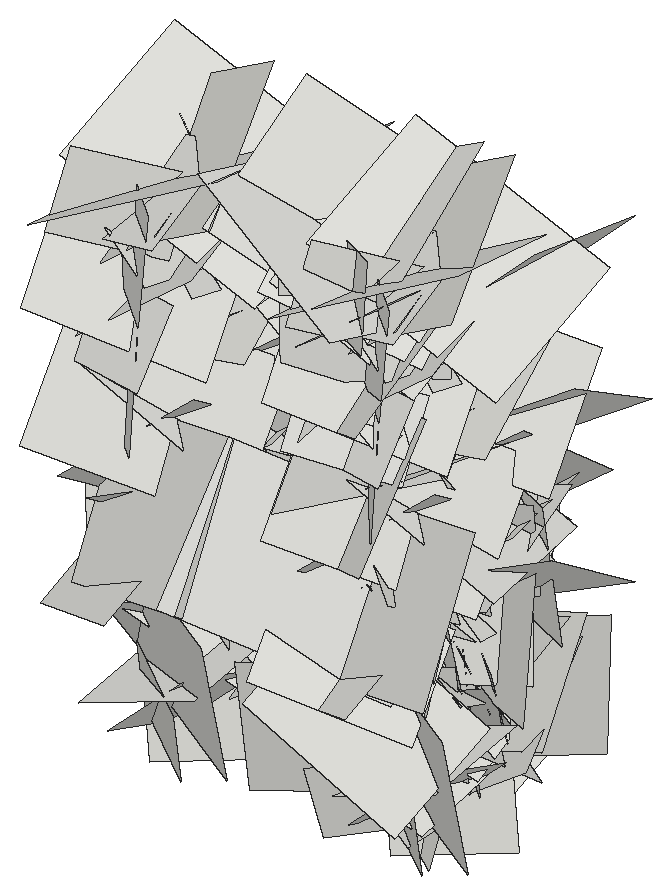
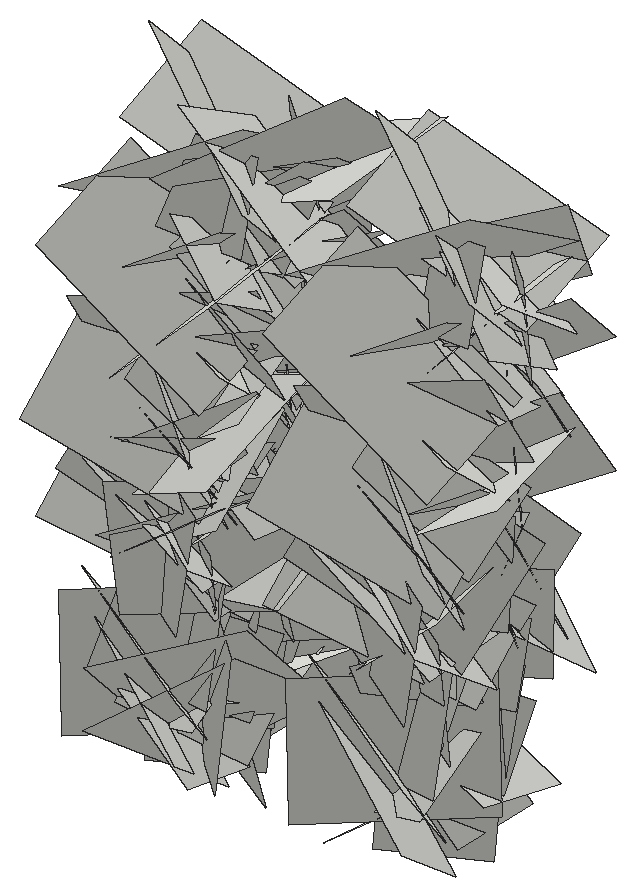
# SketchUp Ruby script. Lengths in inches.
U = 1.inch
M = Sketchup.active_model
def pt(a) = Geom::Point3d.new(a.map { |v| v * U })
def face(e, loops, mat)
  f = e.add_face(loops[0].map { |a| pt(a) })
  loops[1..].each { |l| e.add_face(l.map { |a| pt(a) }).erase! }
  f.material = f.back_material = mat if mat
  f
end
# faces: each face lists its corners as indices into pts; further lists are holes
def faces(e, pts, list, mat = nil) = list.each { |f| face(e, (f[0].is_a?(Array) ? f : [f]).map { |l| l.map { |i| pts[i] } }, mat) }
# xy, xz, yz: faces in a plane at the given z, y or x. An outline is a flat list of corners, or four numbers for a rectangle; further outlines are holes
def ring(l) = l.size == 4 ? [[l[0], l[1]], [l[2], l[1]], [l[2], l[3]], [l[0], l[3]]] : l.each_slice(2).to_a
def flat(e, list, mat, &to3) = list.each { |f| face(e, (f[0].is_a?(Array) ? f : [f]).map { |l| ring(l).map { |u, v| to3.(u, v) } }, mat) }
def xy(e, z, list, mat = nil) = flat(e, list, mat) { |x, y| [x, y, z] }
def xz(e, y, list, mat = nil) = flat(e, list, mat) { |x, z| [x, y, z] }
def yz(e, x, list, mat = nil) = flat(e, list, mat) { |y, z| [x, y, z] }
def lines(e, pts, list) = list.each { |a, b| e.add_line(pt(pts[a]), pt(pts[b])) }
# prism: a flat outline (further loops are holes) pulled along v
def prism(e, loops, v, mat = nil)
  f = face(e, loops, mat); d = Geom::Vector3d.new(v.map { |x| x * U })
  f.pushpull(f.normal.samedirection?(d) ? d.length : -d.length)
end
def box(e, o, s, mat = nil) = prism(e, [[o, [o[0] + s[0], o[1], o[2]], [o[0] + s[0], o[1] + s[1], o[2]], [o[0], o[1] + s[1], o[2]]]], [0, 0, s[2]], mat)
def at(x, y, z, deg = 0) = Geom::Transformation.translation(pt([x, y, z])) * Geom::Transformation.rotation(ORIGIN, Z_AXIS, deg.degrees)
def axes(o, x, y, z) = Geom::Transformation.new([*x, 0, *y, 0, *z, 0, *pt(o).to_a, 1])
def part(name) = M.definitions.add(name)
# library, detail: a bought-in or finely detailed component or shape, given as its bounding box
def library(name, o, s) = part(name).tap { |d| box(d.entities, o, s) }
def detail(e, o, s) = box(e.add_group.entities, o, s)
def put(e, d, t, mat = nil) = e.add_instance(d, t).tap { |i| i.material = mat if mat }
def group(e, t, mat = nil) = e.add_group.tap { |g| g.transformation = t; g.material = mat if mat }.entities
root = M.entities
c1 = part("Component\#6")
p = [[0.01,0,0],[0,3.24,4.54],[4.32,3.24,4.54],[4.33,0,0]]
faces(c1.entities,p,[[0,1,2,3]])
put(root,c1,axes([34.14,170.9375,7.01],[0.11124,0.9843,0.53665],[-0.15751,0.54645,-0.97322],[1.17787,-0.01989,-0.18083]))
put(root,c1,axes([24.34,177.17,11.87],[0.09089,-0.73345,-1.16692],[0.11565,-1.16189,0.73831],[1.45639,0.13804,0.0142]))
put(root,c1,axes([38.11,177.17,11.87],[-0.09089,-0.73345,-1.16692],[-0.11565,-1.16189,0.73831],[-1.45639,0.13804,0.0142]))
put(root,c1,axes([34.14,177.17,11.87],[0.09089,-0.73345,-1.16692],[0.11565,-1.16189,0.73831],[1.45639,0.13804,0.0142]))
put(root,c1,axes([28.31,171.15,7.72],[0.19789,0.75168,0.59634],[-0.00491,0.60823,-0.76521],[-1.01706,0.14332,0.11972]))
put(root,c1,axes([34.14,171.15,7.72],[-0.19789,0.75168,0.59634],[0.00491,0.60823,-0.76521],[1.01706,0.14332,0.11972]))
put(root,c1,axes([38.11,171.15,7.72],[0.19789,0.75168,0.59634],[-0.00491,0.60823,-0.76521],[-1.01706,0.14332,0.11972]))
put(root,c1,axes([28.31,175.79,22.11],[-0.09057,-0.18477,-0.67682],[0.07729,-0.68047,0.17656],[-0.73966,-0.04848,0.10132]))
put(root,c1,axes([34.14,175.79,22.11],[0.09057,-0.18477,-0.67682],[-0.07729,-0.68047,0.17656],[0.73966,-0.04848,0.10132]))
put(root,c1,axes([38.11,175.79,22.11],[-0.09057,-0.18477,-0.67682],[0.07729,-0.68047,0.17656],[-0.73966,-0.04848,0.10132]))
put(root,c1,axes([28.31,172.87,15.39],[0.04258,0.36909,0.59744],[-0.18529,0.58484,-0.34955],[-0.72096,-0.1285,0.12512]))
put(root,c1,axes([34.14,172.87,15.39],[-0.04258,0.36909,0.59744],[0.18529,0.58484,-0.34955],[0.72096,-0.1285,0.12512]))
put(root,c1,axes([38.11,172.87,15.39],[0.04258,0.36909,0.59744],[-0.18529,0.58484,-0.34955],[-0.72096,-0.1285,0.12512]))
put(root,c1,axes([24.34,176.71,20],[0.1716,-1.2405,0.25629],[0.15029,0.2745,1.23906],[1.33426,0.12862,-0.17253]))
put(root,c1,axes([38.11,176.71,20],[-0.1716,-1.2405,0.25629],[-0.15029,0.2745,1.23906],[-1.33426,0.12862,-0.17253]))
put(root,c1,axes([34.14,176.71,20],[0.1716,-1.2405,0.25629],[0.15029,0.2745,1.23906],[1.33426,0.12862,-0.17253]))
put(root,c1,axes([28.31,172.9,17.79],[0.05847,0.04666,0.93522],[0.13105,0.92828,-0.05361],[-0.98388,0.12642,0.04844]))
put(root,c1,axes([34.14,172.9,17.79],[-0.05847,0.04666,0.93522],[-0.13105,0.92828,-0.05361],[0.98388,0.12642,0.04844]))
put(root,c1,axes([38.11,172.9,17.79],[0.05847,0.04666,0.93522],[0.13105,0.92828,-0.05361],[-0.98388,0.12642,0.04844]))
put(root,c1,axes([28.31,172.44,13.26],[-0.14239,0.27787,0.83247],[0.25689,0.82117,-0.23499],[-0.89411,0.19168,-0.20009]))
put(root,c1,axes([34.14,172.44,13.26],[0.14239,0.27787,0.83247],[-0.25689,0.82117,-0.23499],[0.89411,0.19168,-0.20009]))
put(root,c1,axes([38.11,172.44,13.26],[-0.14239,0.27787,0.83247],[0.25689,0.82117,-0.23499],[-0.89411,0.19168,-0.20009]))
put(root,c1,axes([28.31,178.76,18.36],[0.19902,-0.79911,-0.76231],[0.1591,-0.74761,0.82067],[-1.1598,-0.23968,-0.01823]))
put(root,c1,axes([34.14,178.76,18.36],[-0.19902,-0.79911,-0.76231],[-0.1591,-0.74761,0.82067],[1.1598,-0.23968,-0.01823]))
put(root,c1,axes([38.11,178.76,18.36],[0.19902,-0.79911,-0.76231],[0.1591,-0.74761,0.82067],[-1.1598,-0.23968,-0.01823]))
put(root,c1,axes([24.34,178.02,21.625],[-0.10055,-0.80704,-0.57155],[0.14009,-0.57937,0.79615],[1.03886,0.00001,-0.16268]))
put(root,c1,axes([38.11,178.02,21.625],[0.10055,-0.80704,-0.57155],[-0.14009,-0.57937,0.79615],[-1.03886,0.00001,-0.16268]))
put(root,c1,axes([34.14,178.02,21.625],[-0.10055,-0.80704,-0.57155],[0.14009,-0.57937,0.79615],[1.03886,0.00001,-0.16268]))
put(root,c1,axes([24.34,171.875,12.53],[-0.03767,0.74177,1.03266],[-0.14299,1.02503,-0.74093],[1.34014,0.13022,-0.05004]))
put(root,c1,axes([38.11,171.875,12.53],[0.03767,0.74177,1.03266],[0.14299,1.02503,-0.74093],[-1.34014,0.13022,-0.05004]))
put(root,c1,axes([34.14,171.875,12.53],[-0.03767,0.74177,1.03266],[-0.14299,1.02503,-0.74093],[1.34014,0.13022,-0.05004]))
put(root,c1,axes([28.31,176.92,18.36],[-0.03591,-0.7978,0.13647],[0.05211,0.13431,0.79737],[-0.85636,0.04162,0.0428]))
put(root,c1,axes([34.14,176.92,18.36],[0.03591,-0.7978,0.13647],[-0.05211,0.13431,0.79737],[0.85636,0.04162,0.0428]))
put(root,c1,axes([38.11,176.92,18.36],[-0.03591,-0.7978,0.13647],[0.05211,0.13431,0.79737],[-0.85636,0.04162,0.0428]))
put(root,c1,axes([24.34,176.79,7.17],[0.05072,0.23896,-1.1979],[0.10512,-1.19562,-0.23454],[1.29052,0.088,0.06618]))
put(root,c1,axes([38.11,176.79,7.17],[-0.05072,0.23896,-1.1979],[-0.10512,-1.19562,-0.23454],[-1.29052,0.088,0.06618]))
put(root,c1,axes([34.14,176.79,7.17],[0.05072,0.23896,-1.1979],[0.10512,-1.19562,-0.23454],[1.29052,0.088,0.06618]))
put(root,c1,axes([28.31,175.07,0.3],[0.05353,-0.16234,0.63718],[0.01427,0.63917,0.16178],[-0.69684,0.00062,0.05226]))
put(root,c1,axes([34.14,175.07,0.3],[-0.05353,-0.16234,0.63718],[-0.01427,0.63917,0.16178],[0.69684,0.00062,0.05226]))
put(root,c1,axes([38.11,175.07,0.3],[0.05353,-0.16234,0.63718],[0.01427,0.63917,0.16178],[-0.69684,0.00062,0.05226]))
put(root,c1,axes([24.34,178.16,17.01],[0.17232,-1.0163,-0.23365],[-0.0611,-0.24487,1.02499],[1.10369,0.14512,0.09322]))
put(root,c1,axes([38.11,178.16,17.01],[-0.17232,-1.0163,-0.23365],[0.0611,-0.24487,1.02499],[-1.10369,0.14512,0.09322]))
put(root,c1,axes([34.14,178.16,17.01],[0.17232,-1.0163,-0.23365],[-0.0611,-0.24487,1.02499],[1.10369,0.14512,0.09322]))
put(root,c1,axes([24.34,178.75,19.8],[0.0392,-0.90326,-0.49419],[-0.16181,-0.49385,0.89122],[1.07932,-0.04123,0.15156]))
put(root,c1,axes([38.11,178.75,19.8],[-0.0392,-0.90326,-0.49419],[0.16181,-0.49385,0.89122],[-1.07932,-0.04123,0.15156]))
put(root,c1,axes([34.14,178.75,19.8],[0.0392,-0.90326,-0.49419],[-0.16181,-0.49385,0.89122],[1.07932,-0.04123,0.15156]))
put(root,c1,axes([28.31,174.43,8.39],[0.03188,0.26889,0.69876],[-0.00311,0.69936,-0.269],[-0.79363,0.00806,0.02912]))
put(root,c1,axes([34.14,174.43,8.39],[-0.03188,0.26889,0.69876],[0.00311,0.69936,-0.269],[0.79363,0.00806,0.02912]))
put(root,c1,axes([38.11,174.43,8.39],[0.03188,0.26889,0.69876],[-0.00311,0.69936,-0.269],[-0.79363,0.00806,0.02912]))
put(root,c1,axes([24.34,179.79,22.45],[0.18749,-0.99323,-0.93091],[-0.09936,-0.94539,0.99088],[1.43954,0.06411,0.18963]))
put(root,c1,axes([38.11,179.79,22.45],[-0.18749,-0.99323,-0.93091],[0.09936,-0.94539,0.99088],[-1.43954,0.06411,0.18963]))
put(root,c1,axes([34.14,179.79,22.45],[0.18749,-0.99323,-0.93091],[-0.09936,-0.94539,0.99088],[1.43954,0.06411,0.18963]))
put(root,c1,axes([24.34,177.03,8.61],[0.03763,-0.79919,0.49947],[-0.19388,0.48448,0.78821],[0.97999,0.12653,0.13676]))
put(root,c1,axes([38.11,177.03,8.61],[-0.03763,-0.79919,0.49947],[0.19388,0.48448,0.78821],[-0.97999,0.12653,0.13676]))
put(root,c1,axes([34.14,177.03,8.61],[0.03763,-0.79919,0.49947],[-0.19388,0.48448,0.78821],[0.97999,0.12653,0.13676]))
put(root,c1,axes([28.31,177.03,9.04],[0.05145,-0.49737,0.47013],[-0.11624,0.45957,0.49752],[-0.71609,-0.11034,-0.04698]))
put(root,c1,axes([34.14,177.03,9.04],[-0.05145,-0.49737,0.47013],[0.11624,0.45957,0.49752],[0.71609,-0.11034,-0.04698]))
put(root,c1,axes([38.11,177.03,9.04],[0.05145,-0.49737,0.47013],[-0.11624,0.45957,0.49752],[-0.71609,-0.11034,-0.04698]))
put(root,c1,axes([24.34,179.02,2.63],[-0.02304,-0.93672,-0.18796],[0.20199,-0.18848,0.91728],[0.99236,0.01662,-0.19107]))
put(root,c1,axes([38.11,179.02,2.63],[0.02304,-0.93672,-0.18796],[-0.20199,-0.18848,0.91728],[-0.99236,0.01662,-0.19107]))
put(root,c1,axes([34.14,179.02,2.63],[-0.02304,-0.93672,-0.18796],[0.20199,-0.18848,0.91728],[0.99236,0.01662,-0.19107]))
put(root,c1,axes([28.31,175.31,3.87],[0.17194,0.72285,-0.14796],[0.1038,-0.17124,-0.72925],[-0.77519,0.1374,-0.13047]))
put(root,c1,axes([34.14,175.31,3.87],[-0.17194,0.72285,-0.14796],[-0.1038,-0.17124,-0.72925],[0.77519,0.1374,-0.13047]))
put(root,c1,axes([38.11,175.31,3.87],[0.17194,0.72285,-0.14796],[0.1038,-0.17124,-0.72925],[-0.77519,0.1374,-0.13047]))
put(root,c1,axes([24.34,173.88,22.27],[0.13701,1.18016,0.66561],[0.07419,0.66193,-1.18721],[1.4343,-0.14697,-0.00217]))
put(root,c1,axes([38.11,173.88,22.27],[-0.13701,1.18016,0.66561],[-0.07419,0.66193,-1.18721],[-1.4343,-0.14697,-0.00217]))
put(root,c1,axes([34.14,173.88,22.27],[0.13701,1.18016,0.66561],[0.07419,0.66193,-1.18721],[1.4343,-0.14697,-0.00217]))
put(root,c1,axes([24.34,175.28,5.97],[-0.1544,0.17587,1.10387],[0.02973,1.11343,-0.17369],[1.18449,-0.00502,0.14825]))
put(root,c1,axes([38.11,175.28,5.97],[0.1544,0.17587,1.10387],[-0.02973,1.11343,-0.17369],[-1.18449,-0.00502,0.14825]))
put(root,c1,axes([34.14,175.28,5.97],[-0.1544,0.17587,1.10387],[0.02973,1.11343,-0.17369],[1.18449,-0.00502,0.14825]))
put(root,c1,axes([24.34,174.05,15.13],[-0.29087,1.34123,-0.04275],[0.1118,-0.02194,-1.36543],[1.41802,0.27684,0.09888]))
put(root,c1,axes([38.11,174.05,15.13],[0.29087,1.34123,-0.04275],[-0.1118,-0.02194,-1.36543],[-1.41802,0.27684,0.09888]))
put(root,c1,axes([34.14,174.05,15.13],[-0.29087,1.34123,-0.04275],[0.1118,-0.02194,-1.36543],[1.41802,0.27684,0.09888]))
put(root,c1,axes([24.34,177.91,2.6],[0.0759,-0.493,0.60539],[0.11612,0.60826,0.48238],[0.8194,-0.04053,-0.12444]))
put(root,c1,axes([38.11,177.91,2.6],[-0.0759,-0.493,0.60539],[-0.11612,0.60826,0.48238],[-0.8194,-0.04053,-0.12444]))
put(root,c1,axes([34.14,177.91,2.6],[0.0759,-0.493,0.60539],[0.11612,0.60826,0.48238],[0.8194,-0.04053,-0.12444]))
put(root,c1,axes([28.31,179.07,16.9375],[-0.01654,-0.76992,0.15337],[0.18248,0.14631,0.752],[-0.8119,0.04857,0.16589]))
put(root,c1,axes([34.14,179.07,16.9375],[0.01654,-0.76992,0.15337],[-0.18248,0.14631,0.752],[0.8119,0.04857,0.16589]))
put(root,c1,axes([38.11,179.07,16.9375],[-0.01654,-0.76992,0.15337],[0.18248,0.14631,0.752],[-0.8119,0.04857,0.16589]))
put(root,c1,axes([24.34,177.25,5.58],[0.00826,-0.19404,0.73725],[0.12542,0.72866,0.19053],[0.79831,-0.11247,-0.03756]))
put(root,c1,axes([38.11,177.25,5.58],[-0.00826,-0.19404,0.73725],[-0.12542,0.72866,0.19053],[-0.79831,-0.11247,-0.03756]))
put(root,c1,axes([34.14,177.25,5.58],[0.00826,-0.19404,0.73725],[0.12542,0.72866,0.19053],[0.79831,-0.11247,-0.03756]))
put(root,c1,axes([28.31,178.9,4.98],[0.12785,-0.58421,0.25103],[-0.01096,0.25367,0.59532],[-0.67392,-0.11496,0.03794]))
put(root,c1,axes([34.14,178.9,4.98],[-0.12785,-0.58421,0.25103],[0.01096,0.25367,0.59532],[0.67392,-0.11496,0.03794]))
put(root,c1,axes([38.11,178.9,4.98],[0.12785,-0.58421,0.25103],[-0.01096,0.25367,0.59532],[-0.67392,-0.11496,0.03794]))
put(root,c1,axes([28.31,177.55,19],[0.11507,-0.3549,0.71119],[0.00206,0.71791,0.35796],[-0.84251,-0.04671,0.09801]))
put(root,c1,axes([34.14,177.55,19],[-0.11507,-0.3549,0.71119],[-0.00206,0.71791,0.35796],[0.84251,-0.04671,0.09801]))
put(root,c1,axes([38.11,177.55,19],[0.11507,-0.3549,0.71119],[0.00206,0.71791,0.35796],[-0.84251,-0.04671,0.09801]))
put(root,c1,axes([24.34,179.43,6.59],[0.14458,-1.15784,0.73248],[0.20973,0.74503,1.14083],[1.43706,0.00775,-0.24019]))
put(root,c1,axes([38.11,179.43,6.59],[-0.14458,-1.15784,0.73248],[-0.20973,0.74503,1.14083],[-1.43706,0.00775,-0.24019]))
put(root,c1,axes([34.14,179.43,6.59],[0.14458,-1.15784,0.73248],[0.20973,0.74503,1.14083],[1.43706,0.00775,-0.24019]))
put(root,c1,axes([24.34,177.67,8.79],[0.10774,-0.22129,0.90038],[0.20078,0.89162,0.19775],[0.96207,-0.1613,-0.1421]))
put(root,c1,axes([38.11,177.67,8.79],[-0.10774,-0.22129,0.90038],[-0.20078,0.89162,0.19775],[-0.96207,-0.1613,-0.1421]))
put(root,c1,axes([34.14,177.67,8.79],[0.10774,-0.22129,0.90038],[0.20078,0.89162,0.19775],[0.96207,-0.1613,-0.1421]))
put(root,c1,axes([28.31,179.66,2.51],[0.14219,-0.09473,-0.68692],[-0.01318,-0.69988,0.09409],[-0.73491,-0.00578,-0.13459]))
put(root,c1,axes([34.14,179.66,2.51],[-0.14219,-0.09473,-0.68692],[0.01318,-0.69988,0.09409],[0.73491,-0.00578,-0.13459]))
put(root,c1,axes([38.11,179.66,2.51],[0.14219,-0.09473,-0.68692],[-0.01318,-0.69988,0.09409],[-0.73491,-0.00578,-0.13459]))
put(root,c1,axes([28.31,180.59,3.91],[0.10883,-0.74668,-0.23347],[-0.0349,-0.23939,0.75113],[-0.82853,-0.08799,-0.06231]))
put(root,c1,axes([34.14,180.59,3.91],[-0.10883,-0.74668,-0.23347],[0.0349,-0.23939,0.75113],[0.82853,-0.08799,-0.06231]))
put(root,c1,axes([38.11,180.59,3.91],[0.10883,-0.74668,-0.23347],[-0.0349,-0.23939,0.75113],[-0.82853,-0.08799,-0.06231]))
put(root,c1,axes([28.31,180.83,12.7],[0.12371,-0.65209,-0.45157],[0.04757,-0.45027,0.66181],[-0.83942,-0.12162,-0.02905]))
put(root,c1,axes([34.14,180.83,12.7],[-0.12371,-0.65209,-0.45157],[-0.04757,-0.45027,0.66181],[0.83942,-0.12162,-0.02905]))
put(root,c1,axes([38.11,180.83,12.7],[0.12371,-0.65209,-0.45157],[0.04757,-0.45027,0.66181],[-0.83942,-0.12162,-0.02905]))
put(root,c1,axes([24.34,180.99,16.6875],[0.01817,-0.80344,-0.66577],[0.22863,-0.64876,0.78846],[1.08217,0.15055,-0.1554]))
put(root,c1,axes([38.11,180.99,16.6875],[-0.01817,-0.80344,-0.66577],[-0.22863,-0.64876,0.78846],[-1.08217,0.15055,-0.1554]))
put(root,c1,axes([34.14,180.99,16.6875],[0.01817,-0.80344,-0.66577],[0.22863,-0.64876,0.78846],[1.08217,0.15055,-0.1554]))
put(root,c1,axes([24.34,176.29,14.82],[0.00549,0.62123,1.00169],[0.24363,0.98194,-0.61017],[1.22543,-0.19801,0.11682]))
put(root,c1,axes([38.11,176.29,14.82],[-0.00549,0.62123,1.00169],[-0.24363,0.98194,-0.61017],[-1.22543,-0.19801,0.11682]))
put(root,c1,axes([34.14,176.29,14.82],[0.00549,0.62123,1.00169],[0.24363,0.98194,-0.61017],[1.22543,-0.19801,0.11682]))
put(root,c1,axes([28.31,178.54,4.68],[-0.06155,-0.26232,0.60589],[-0.0363,0.6086,0.26022],[-0.69891,-0.00851,-0.06687]))
put(root,c1,axes([34.14,178.54,4.68],[0.06155,-0.26232,0.60589],[0.0363,0.6086,0.26022],[0.69891,-0.00851,-0.06687]))
put(root,c1,axes([38.11,178.54,4.68],[-0.06155,-0.26232,0.60589],[-0.0363,0.6086,0.26022],[-0.69891,-0.00851,-0.06687]))
put(root,c1,axes([38.11,179.8125,11.71],[-0.00414,-0.7832,0.49624],[0.01003,0.49619,0.78318],[-0.98275,0.00836,0.0059]))
put(root,c1,axes([24.34,179.8125,11.71],[0.00414,-0.7832,0.49624],[-0.01003,0.49619,0.78318],[0.98275,0.00836,0.0059]))
put(root,c1,axes([34.14,179.8125,11.71],[0.00414,-0.7832,0.49624],[-0.01003,0.49619,0.78318],[0.98275,0.00836,0.0059]))
put(root,c1,axes([24.34,181.49,10.05],[0.07357,-0.24485,-1.22332],[0.09578,-1.221,0.24951],[1.31896,0.10233,0.05011]))
put(root,c1,axes([38.11,181.49,10.05],[-0.07357,-0.24485,-1.22332],[-0.09578,-1.221,0.24951],[-1.31896,0.10233,0.05011]))
put(root,c1,axes([34.14,181.49,10.05],[0.07357,-0.24485,-1.22332],[0.09578,-1.221,0.24951],[1.31896,0.10233,0.05011]))
put(root,c1,axes([28.31,181.21,19.66],[0.0984,-0.57654,-0.29954],[0.01889,-0.30021,0.58335],[-0.68843,-0.09064,-0.02681]))
put(root,c1,axes([34.14,181.21,19.66],[-0.0984,-0.57654,-0.29954],[-0.01889,-0.30021,0.58335],[0.68843,-0.09064,-0.02681]))
put(root,c1,axes([38.11,181.21,19.66],[0.0984,-0.57654,-0.29954],[0.01889,-0.30021,0.58335],[-0.68843,-0.09064,-0.02681]))
put(root,c1,axes([28.31,181.24,7.39],[0.09835,-0.8461,0.11424],[0.10744,0.12502,0.84359],[-0.89861,-0.07766,0.11336]))
put(root,c1,axes([34.14,181.24,7.39],[-0.09835,-0.8461,0.11424],[-0.10744,0.12502,0.84359],[0.89861,-0.07766,0.11336]))
put(root,c1,axes([38.11,181.24,7.39],[0.09835,-0.8461,0.11424],[0.10744,0.12502,0.84359],[-0.89861,-0.07766,0.11336]))
put(root,c1,axes([24.34,180.26,8.26],[-0.04265,-1.00211,0.75475],[-0.17142,0.75298,0.99114],[1.31872,0.06547,0.15325]))
put(root,c1,axes([38.11,180.26,8.26],[0.04265,-1.00211,0.75475],[0.17142,0.75298,0.99114],[-1.31872,0.06547,0.15325]))
put(root,c1,axes([34.14,180.26,8.26],[-0.04265,-1.00211,0.75475],[-0.17142,0.75298,0.99114],[1.31872,0.06547,0.15325]))
put(root,c1,axes([24.34,182.69,9.96],[-0.0402,-0.96504,-0.67279],[0.04089,-0.67379,0.96431],[1.24632,-0.00902,-0.05333]))
put(root,c1,axes([38.11,182.69,9.96],[0.0402,-0.96504,-0.67279],[-0.04089,-0.67379,0.96431],[-1.24632,-0.00902,-0.05333]))
put(root,c1,axes([34.14,182.69,9.96],[-0.0402,-0.96504,-0.67279],[0.04089,-0.67379,0.96431],[1.24632,-0.00902,-0.05333]))
put(root,c1,axes([24.34,182.3,13.14],[0.06012,-0.59744,-0.78978],[-0.12867,-0.78931,0.58836],[1.0418,-0.06301,0.11824]))
put(root,c1,axes([38.11,182.3,13.14],[-0.06012,-0.59744,-0.78978],[0.12867,-0.78931,0.58836],[-1.0418,-0.06301,0.11824]))
put(root,c1,axes([34.14,182.3,13.14],[0.06012,-0.59744,-0.78978],[-0.12867,-0.78931,0.58836],[1.0418,-0.06301,0.11824]))
put(root,c1,axes([28.31,181.23,7.68],[-0.09173,-0.20092,-0.6203],[0.07215,-0.6251,0.19298],[-0.68737,-0.0388,0.10304]))
put(root,c1,axes([34.14,181.23,7.68],[0.09173,-0.20092,-0.6203],[-0.07215,-0.6251,0.19298],[0.68737,-0.0388,0.10304]))
put(root,c1,axes([38.11,181.23,7.68],[-0.09173,-0.20092,-0.6203],[0.07215,-0.6251,0.19298],[-0.68737,-0.0388,0.10304]))
put(root,c1,axes([24.34,179.12,5.58],[0.07323,0.67973,-0.51678],[0.08286,-0.52133,-0.67526],[0.90131,-0.0073,0.10406]))
put(root,c1,axes([38.11,179.12,5.58],[-0.07323,0.67973,-0.51678],[-0.08286,-0.52133,-0.67526],[-0.90131,-0.0073,0.10406]))
put(root,c1,axes([34.14,179.12,5.58],[0.07323,0.67973,-0.51678],[0.08286,-0.52133,-0.67526],[0.90131,-0.0073,0.10406]))
put(root,c1,axes([24.34,181.89,8.77],[0.15486,-1.04414,-0.08659],[-0.04063,-0.0927,1.0531],[1.10985,0.1423,0.05063]))
put(root,c1,axes([38.11,181.89,8.77],[-0.15486,-1.04414,-0.08659],[0.04063,-0.0927,1.0531],[-1.10985,0.1423,0.05063]))
put(root,c1,axes([34.14,181.89,8.77],[0.15486,-1.04414,-0.08659],[-0.04063,-0.0927,1.0531],[1.10985,0.1423,0.05063]))
put(root,c1,axes([24.34,182.08,15.67],[0.13861,-1.35642,0.31459],[-0.2886,0.28497,1.34186],[1.44748,0.1867,0.23742]))
put(root,c1,axes([38.11,182.08,15.67],[-0.13861,-1.35642,0.31459],[0.2886,0.28497,1.34186],[-1.44748,0.1867,0.23742]))
put(root,c1,axes([34.14,182.08,15.67],[0.13861,-1.35642,0.31459],[-0.2886,0.28497,1.34186],[1.44748,0.1867,0.23742]))
put(root,c1,axes([38.11,180.69,8.55],[0.12889,0.40226,-0.91097],[0.04748,-0.91901,-0.39983],[-1.05451,0.00779,-0.12935]))
put(root,c1,axes([24.34,180.69,8.55],[-0.12889,0.40226,-0.91097],[-0.04748,-0.91901,-0.39983],[1.05451,0.00779,-0.12935]))
put(root,c1,axes([34.14,180.69,8.55],[-0.12889,0.40226,-0.91097],[-0.04748,-0.91901,-0.39983],[1.05451,0.00779,-0.12935]))
put(root,c1,axes([24.34,178.03,1.86],[0.09591,-0.07879,1.2407],[-0.19288,1.22975,0.09137],[1.3036,0.18775,-0.07776]))
put(root,c1,axes([38.11,178.03,1.86],[-0.09591,-0.07879,1.2407],[0.19288,1.22975,0.09137],[-1.3036,0.18775,-0.07776]))
put(root,c1,axes([34.14,178.03,1.86],[0.09591,-0.07879,1.2407],[-0.19288,1.22975,0.09137],[1.3036,0.18775,-0.07776]))
put(root,c1,axes([28.31,178.57,11.38],[0.09025,0.42259,0.64735],[-0.15778,0.64804,-0.40347],[-0.80413,-0.07973,0.15182]))
put(root,c1,axes([34.14,178.57,11.38],[-0.09025,0.42259,0.64735],[0.15778,0.64804,-0.40347],[0.80413,-0.07973,0.15182]))
put(root,c1,axes([38.11,178.57,11.38],[0.09025,0.42259,0.64735],[-0.15778,0.64804,-0.40347],[-0.80413,-0.07973,0.15182]))
put(root,c1,axes([24.34,181.48,10.98],[0.16941,-1.10786,0.62997],[-0.04307,0.63015,1.11849],[1.35023,0.1591,-0.04336]))
put(root,c1,axes([38.11,181.48,10.98],[-0.16941,-1.10786,0.62997],[0.04307,0.63015,1.11849],[-1.35023,0.1591,-0.04336]))
put(root,c1,axes([34.14,181.48,10.98],[0.16941,-1.10786,0.62997],[-0.04307,0.63015,1.11849],[1.35023,0.1591,-0.04336]))
put(root,c1,axes([24.34,183.39,2.71],[0.21072,-0.93049,-0.66529],[-0.0846,-0.6849,0.93407],[1.20954,0.1142,0.18123]))
put(root,c1,axes([38.11,183.39,2.71],[-0.21072,-0.93049,-0.66529],[0.0846,-0.6849,0.93407],[-1.20954,0.1142,0.18123]))
put(root,c1,axes([34.14,183.39,2.71],[0.21072,-0.93049,-0.66529],[-0.0846,-0.6849,0.93407],[1.20954,0.1142,0.18123]))
put(root,c1,axes([24.34,182.3,11.84],[0.17648,0.01407,-1.1199],[0.09677,-1.12861,-0.00061],[1.18323,0.09021,0.16708]))
put(root,c1,axes([38.11,182.3,11.84],[-0.17648,0.01407,-1.1199],[-0.09677,-1.12861,-0.00061],[-1.18323,0.09021,0.16708]))
put(root,c1,axes([34.14,182.3,11.84],[0.17648,0.01407,-1.1199],[0.09677,-1.12861,-0.00061],[1.18323,0.09021,0.16708]))
put(root,c1,axes([24.34,183.3125,5.12],[0.15127,-0.71846,-0.81538],[0.11003,-0.80961,0.73154],[1.14669,0.17246,0.03737]))
put(root,c1,axes([38.11,183.3125,5.12],[-0.15127,-0.71846,-0.81538],[-0.11003,-0.80961,0.73154],[-1.14669,0.17246,0.03737]))
put(root,c1,axes([34.14,183.3125,5.12],[0.15127,-0.71846,-0.81538],[0.11003,-0.80961,0.73154],[1.14669,0.17246,0.03737]))
put(root,c1,axes([28.31,182.67,1.51],[0.02969,-0.72745,-0.10184],[0.03667,-0.1005,0.72735],[-0.77775,-0.03251,0.03041]))
put(root,c1,axes([34.14,182.67,1.51],[-0.02969,-0.72745,-0.10184],[-0.03667,-0.1005,0.72735],[0.77775,-0.03251,0.03041]))
